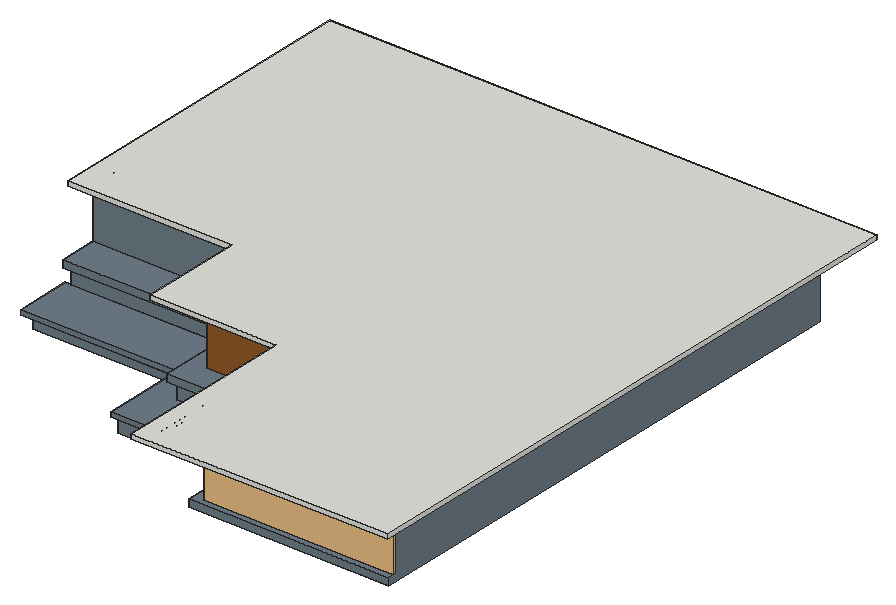
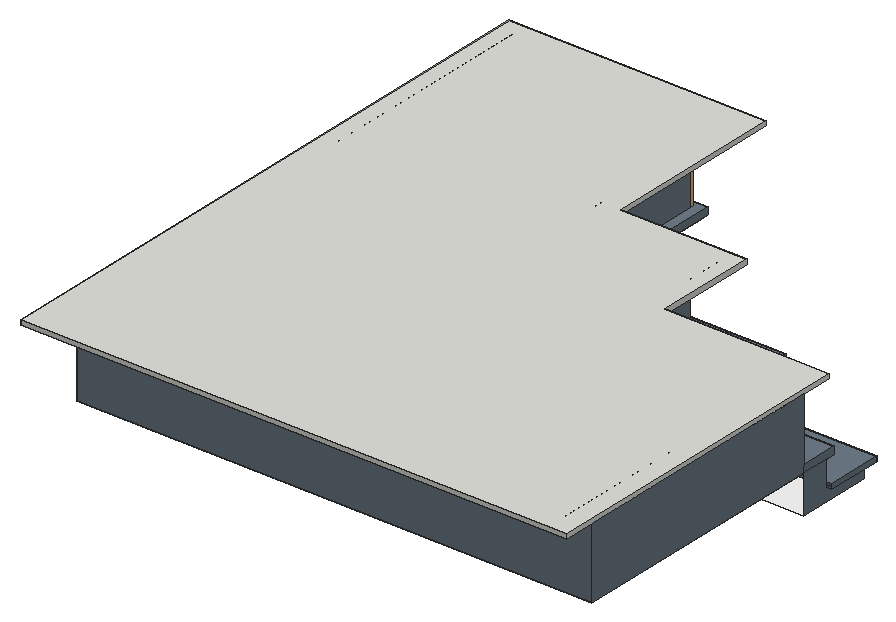
# SketchUp Ruby script. Lengths in inches.
U = 1.inch
M = Sketchup.active_model
def pt(a) = Geom::Point3d.new(a.map { |v| v * U })
def face(e, loops, mat)
  f = e.add_face(loops[0].map { |a| pt(a) })
  loops[1..].each { |l| e.add_face(l.map { |a| pt(a) }).erase! }
  f.material = f.back_material = mat if mat
  f
end
# faces: each face lists its corners as indices into pts; further lists are holes
def faces(e, pts, list, mat = nil) = list.each { |f| face(e, (f[0].is_a?(Array) ? f : [f]).map { |l| l.map { |i| pts[i] } }, mat) }
# xy, xz, yz: faces in a plane at the given z, y or x. An outline is a flat list of corners, or four numbers for a rectangle; further outlines are holes
def ring(l) = l.size == 4 ? [[l[0], l[1]], [l[2], l[1]], [l[2], l[3]], [l[0], l[3]]] : l.each_slice(2).to_a
def flat(e, list, mat, &to3) = list.each { |f| face(e, (f[0].is_a?(Array) ? f : [f]).map { |l| ring(l).map { |u, v| to3.(u, v) } }, mat) }
def xy(e, z, list, mat = nil) = flat(e, list, mat) { |x, y| [x, y, z] }
def xz(e, y, list, mat = nil) = flat(e, list, mat) { |x, z| [x, y, z] }
def yz(e, x, list, mat = nil) = flat(e, list, mat) { |y, z| [x, y, z] }
def lines(e, pts, list) = list.each { |a, b| e.add_line(pt(pts[a]), pt(pts[b])) }
# prism: a flat outline (further loops are holes) pulled along v
def prism(e, loops, v, mat = nil)
  f = face(e, loops, mat); d = Geom::Vector3d.new(v.map { |x| x * U })
  f.pushpull(f.normal.samedirection?(d) ? d.length : -d.length)
end
def box(e, o, s, mat = nil) = prism(e, [[o, [o[0] + s[0], o[1], o[2]], [o[0] + s[0], o[1] + s[1], o[2]], [o[0], o[1] + s[1], o[2]]]], [0, 0, s[2]], mat)
def at(x, y, z, deg = 0) = Geom::Transformation.translation(pt([x, y, z])) * Geom::Transformation.rotation(ORIGIN, Z_AXIS, deg.degrees)
def axes(o, x, y, z) = Geom::Transformation.new([*x, 0, *y, 0, *z, 0, *pt(o).to_a, 1])
def part(name) = M.definitions.add(name)
# library, detail: a bought-in or finely detailed component or shape, given as its bounding box
def library(name, o, s) = part(name).tap { |d| box(d.entities, o, s) }
def detail(e, o, s) = box(e.add_group.entities, o, s)
def put(e, d, t, mat = nil) = e.add_instance(d, t).tap { |i| i.material = mat if mat }
def group(e, t, mat = nil) = e.add_group.tap { |g| g.transformation = t; g.material = mat if mat }.entities
root = M.entities
M.materials.add("Heather_Cuffs").color = [111, 126, 137]
M.materials.add("[Color E05]").color = [255, 255, 0]
M.materials.add("[Color M00]").color = [255, 255, 255]
M.materials.add("[Color M01]").color = [226, 226, 226]
M.materials.add("[Wood Cherry Original]").color = [152, 86, 42]
M.materials.add("[Wood Floor Parquet]").color = [145, 89, 39]
M.materials.add("termopan").color = [253, 253, 253]
c1 = library("Fence panel",[0,-3,0],[162,3,54])
xy(root,330,[[490.93,297.91,490.15,298.01,489.43,298.31,488.81,298.79,488.33,299.41,488.03,300.13,487.93,300.91,488.03,301.68,488.33,302.41,488.81,303.03,489.43,303.5,490.15,303.8,490.93,303.91,491.71,303.8,492.43,303.5,493.05,303.03,493.53,302.41,493.83,301.68,493.93,300.91,493.83,300.13,493.53,299.41,493.05,298.79,492.43,298.31,491.71,298.01],[406.58,298.81,405.81,298.91,405.08,299.21,404.46,299.69,403.98,300.31,403.69,301.03,403.58,301.81,403.69,302.58,403.98,303.31,404.46,303.93,405.08,304.4,405.81,304.7,406.58,304.81,407.36,304.7,408.08,304.4,408.7,303.93,409.18,303.31,409.48,302.58,409.58,301.81,409.48,301.03,409.18,300.31,408.7,299.69,408.08,299.21,407.36,298.91],[300.21,365.29,299.43,365.39,298.71,365.69,298.09,366.17,297.61,366.79,297.3125,367.52,297.21,368.29,297.3125,369.07,297.61,369.79,298.09,370.41,298.71,370.89,299.43,371.19,300.21,371.29,300.99,371.19,301.71,370.89,302.33,370.41,302.81,369.79,303.11,369.07,303.21,368.29,303.11,367.52,302.81,366.79,302.33,366.17,301.71,365.69,300.99,365.39],[338.49,366.3,337.71,366.4,336.99,366.7,336.37,367.18,335.89,367.8,335.59,368.52,335.49,369.3,335.59,370.08,335.89,370.8,336.37,371.42,336.99,371.9,337.71,372.2,338.49,372.3,339.27,372.2,339.99,371.9,340.61,371.42,341.09,370.8,341.39,370.08,341.49,369.3,341.39,368.52,341.09,367.8,340.61,367.18,339.99,366.7,339.27,366.4],[372.37,366.74,371.59,366.84,370.87,367.14,370.25,367.62,369.77,368.24,369.47,368.96,369.37,369.74,369.47,370.51,369.77,371.24,370.25,371.86,370.87,372.34,371.59,372.63,372.37,372.74,373.15,372.63,373.87,372.34,374.49,371.86,374.97,371.24,375.27,370.51,375.37,369.74,375.27,368.96,374.97,368.24,374.49,367.62,373.87,367.14,373.15,366.84]],"[Color E05]")
xy(root,331,[[[395.22,281.96,395.22,356.89,262.22,356.89,262.22,420.96,429.22,420.96,429.22,333.96,540.22,333.96,540.22,281.96],[490.93,297.91,491.71,298.01,492.43,298.31,493.05,298.79,493.53,299.41,493.83,300.13,493.93,300.91,493.83,301.68,493.53,302.41,493.05,303.03,492.43,303.5,491.71,303.8,490.93,303.91,490.15,303.8,489.43,303.5,488.81,303.03,488.33,302.41,488.03,301.68,487.93,300.91,488.03,300.13,488.33,299.41,488.81,298.79,489.43,298.31,490.15,298.01],[300.21,365.29,300.99,365.39,301.71,365.69,302.33,366.17,302.81,366.79,303.11,367.52,303.21,368.29,303.11,369.07,302.81,369.79,302.33,370.41,301.71,370.89,300.99,371.19,300.21,371.29,299.43,371.19,298.71,370.89,298.09,370.41,297.61,369.79,297.3125,369.07,297.21,368.29,297.3125,367.52,297.61,366.79,298.09,366.17,298.71,365.69,299.43,365.39],[338.49,366.3,339.27,366.4,339.99,366.7,340.61,367.18,341.09,367.8,341.39,368.52,341.49,369.3,341.39,370.08,341.09,370.8,340.61,371.42,339.99,371.9,339.27,372.2,338.49,372.3,337.71,372.2,336.99,371.9,336.37,371.42,335.89,370.8,335.59,370.08,335.49,369.3,335.59,368.52,335.89,367.8,336.37,367.18,336.99,366.7,337.71,366.4],[372.37,366.74,373.15,366.84,373.87,367.14,374.49,367.62,374.97,368.24,375.27,368.96,375.37,369.74,375.27,370.51,374.97,371.24,374.49,371.86,373.87,372.34,373.15,372.63,372.37,372.74,371.59,372.63,370.87,372.34,370.25,371.86,369.77,371.24,369.47,370.51,369.37,369.74,369.47,368.96,369.77,368.24,370.25,367.62,370.87,367.14,371.59,366.84],[406.58,298.81,407.36,298.91,408.08,299.21,408.7,299.69,409.18,300.31,409.48,301.03,409.58,301.81,409.48,302.58,409.18,303.31,408.7,303.93,408.08,304.4,407.36,304.7,406.58,304.81,405.81,304.7,405.08,304.4,404.46,303.93,403.98,303.31,403.69,302.58,403.58,301.81,403.69,301.03,403.98,300.31,404.46,299.69,405.08,299.21,405.81,298.91]]],"termopan")
xy(root,343,[[391.22,278.96,415.22,281.96],[415.22,278.96,540.22,281.96],[391.22,281.96,395.22,319.96],[395.22,281.96,415.22,319.96],[415.22,281.96,540.22,319.96],
  [395.22,319.96,415.22,319.96,415.22,397.89,413.22,397.89,413.22,395.89,262.22,395.89,262.22,356.89,395.22,356.89],[391.22,319.96,395.22,356.89],[257.22,349.89,262.22,395.89],[262.22,349.89,391.22,356.89],[257.22,395.89,262.22,397.89],
  [262.22,395.89,402.22,397.89],[402.22,395.89,413.22,397.89]],"Heather_Cuffs")
xy(root,347,[[391.22,278.96,540.22,278.96,540.22,319.96,415.22,319.96,415.22,397.89,257.22,397.89,257.22,349.89,391.22,349.89]],"Heather_Cuffs")
xy(root,363.8,[[531.22,186.96,702.22,194.96],[[540.22,194.96,702.22,194.96,702.22,646.96,262.22,646.96,262.22,397.89,415.22,397.89,415.22,319.96,540.22,319.96],[549.22,203.96,549.22,342.96,438.22,342.96,438.22,429.96,271.22,429.96,271.22,637.96,693.22,637.96,693.22,203.96]],[531.22,194.96,540.22,278.96],[531.22,278.96,540.22,281.96],[531.22,281.96,540.22,319.96],
  [413.22,310.96,531.22,319.96],[413.22,319.96,415.22,397.89],[262.22,388.89,402.22,397.89],[402.22,388.89,413.22,397.89]],"Heather_Cuffs")
xy(root,370,[[531.22,186.96,702.22,186.96,702.22,194.96,540.22,194.96,540.22,333.96,429.22,333.96,429.22,420.96,262.22,420.96,262.22,388.89,413.22,388.89,413.22,310.96,531.22,310.96],[438.22,342.96,438.35,420.96]],"Heather_Cuffs")
xy(root,424,[[540.22,194.96,702.22,194.96,702.22,646.96,262.22,646.96,262.22,420.96,429.22,420.96,429.22,333.96,549.22,333.96,549.22,342.96,438.35,342.96,438.35,420.96,438.22,420.96,438.22,429.96,271.22,429.96,271.22,637.96,693.22,637.96,693.22,203.96,549.22,203.96,549.22,333.96,540.22,333.96]],"Heather_Cuffs")
xy(root,424,[[[510.22,151.96,510.22,306.96,402.22,306.96,402.22,393.96,262.22,393.96,262.22,673.96,729.22,673.96,729.22,151.96],[523.35,165.08,716.09,165.08,716.09,660.83,275.35,660.83,275.35,407.08,415.35,407.08,415.35,320.08,523.35,320.08]],[526.88,168.61,526.88,323.61,418.88,323.61,418.88,410.61,278.88,410.61,278.88,657.3,712.5625,657.3,712.5625,168.61]],"[Wood Cherry Original]")
xy(root,427,[[[523.35,165.08,523.35,320.08,415.35,320.08,415.35,407.08,275.35,407.08,275.35,660.83,716.09,660.83,716.09,165.08],[526.88,168.61,712.5625,168.61,712.5625,657.3,278.88,657.3,278.88,410.61,418.88,410.61,418.88,323.61,526.88,323.61]]],"[Color E05]")
xy(root,428,[[510.22,151.96,729.22,151.96,729.22,673.96,262.22,673.96,262.22,393.96,402.22,393.96,402.22,306.96,510.22,306.96]])
xz(root,151.96,[[510.22,424,729.22,428]])
xz(root,165.08,[[523.35,424,716.09,427]])
xz(root,168.61,[[526.88,424,712.5625,427]])
xz(root,186.96,[[531.22,363.8,702.22,370]],"Heather_Cuffs")
xz(root,194.96,[[543.35,370,693.22,424],[693.22,370,702.22,424]],"Heather_Cuffs")
xz(root,203.96,[[549.22,363.8,693.22,424]],"Heather_Cuffs")
xz(root,278.96,[[391.22,343,540.22,347]],"Heather_Cuffs")
xz(root,281.96,[[395.22,331,540.22,343]],"Heather_Cuffs")
xz(root,306.96,[[402.22,424,510.22,428]])
xz(root,310.96,[[413.22,363.8,531.22,370]],"Heather_Cuffs")
xz(root,319.96,[[415.22,343,540.22,347],[415.22,347,540.22,363.8]],"Heather_Cuffs")
xz(root,320.08,[[415.35,424,523.35,427]])
xz(root,323.61,[[418.88,424,526.88,427]])
xz(root,333.96,[[540.22,370,540.22,424,549.22,424]],"Heather_Cuffs")
xz(root,333.96,[[429.22,370,540.22,424]],"[Wood Floor Parquet]")
xz(root,342.96,[[438.22,363.8,438.22,370,438.35,370,438.35,424,549.22,424,549.22,363.8]],"Heather_Cuffs")
xz(root,349.89,[[257.22,343,391.22,347]],"Heather_Cuffs")
xz(root,356.89,[[262.22,331,395.22,343]],"Heather_Cuffs")
xz(root,388.89,[[262.22,363.8,413.22,370]],"Heather_Cuffs")
xz(root,393.96,[[262.22,424,402.22,428]])
xz(root,397.89,[[257.22,343,262.22,345],[262.22,343,402.22,347],[402.22,343,413.22,347],[413.22,343,415.22,347],[257.22,345,262.22,347],
  [262.22,347,402.22,363.8],[402.22,347,413.22,363.8],[413.22,347,415.22,363.8]],"Heather_Cuffs")
xz(root,407.08,[[275.35,424,415.35,427]])
xz(root,410.61,[[278.88,424,418.88,427]])
xz(root,420.96,[[262.22,370,429.22,424],[438.22,370,438.35,424]],"Heather_Cuffs")
xz(root,429.96,[[271.22,363.8,438.22,424]],"Heather_Cuffs")
xz(root,637.96,[[271.22,363.8,693.22,424]],"Heather_Cuffs")
xz(root,646.96,[[262.22,363.8,702.22,424]],"Heather_Cuffs")
xz(root,657.3,[[278.88,424,712.5625,427]])
xz(root,660.83,[[275.35,424,716.09,427]])
xz(root,673.96,[[262.22,424,729.22,428]])
yz(root,257.22,[[349.89,343,397.89,347]],"Heather_Cuffs")
yz(root,262.22,[[393.96,424,673.96,428]])
yz(root,262.22,[[356.89,331,356.89,343,397.89,343,397.89,363.8,420.96,363.8,420.96,331],[388.89,363.8,420.96,370],[420.96,363.8,646.96,424]],"Heather_Cuffs")
yz(root,271.22,[[429.96,363.8,637.96,424]],"Heather_Cuffs")
yz(root,275.35,[[407.08,424,660.83,427]])
yz(root,278.88,[[410.61,424,657.3,427]])
yz(root,391.22,[[278.96,343,349.89,347]],"Heather_Cuffs")
yz(root,395.22,[[281.96,331,356.89,343]],"Heather_Cuffs")
yz(root,402.22,[[306.96,424,393.96,428]])
yz(root,413.22,[[395.89,343,397.89,345],[310.96,363.8,388.89,370]],"Heather_Cuffs")
yz(root,415.22,[[319.96,343,397.89,347],[319.96,347,397.89,363.8]],"Heather_Cuffs")
yz(root,415.35,[[320.08,424,407.08,427]])
yz(root,418.88,[[323.61,424,410.61,427]])
yz(root,429.22,[[333.96,370,420.96,424]],"Heather_Cuffs")
yz(root,438.22,[[342.96,363.8,429.96,363.8,429.96,424,420.96,424,420.96,370,342.96,370]],"Heather_Cuffs")
yz(root,438.35,[[342.96,370,420.96,424]],"Heather_Cuffs")
yz(root,510.22,[[151.96,424,306.96,428]])
yz(root,523.35,[[165.08,424,320.08,427]])
yz(root,526.88,[[168.61,424,323.61,427]])
yz(root,531.22,[[186.96,363.8,310.96,370]],"Heather_Cuffs")
yz(root,540.22,[[278.96,343,281.96,347],[281.96,343,319.96,347],[278.96,347,281.96,363.8],[281.96,347,319.96,363.8],[194.96,370,333.96,424]],"Heather_Cuffs")
yz(root,549.22,[[203.96,363.8,342.96,424]],"Heather_Cuffs")
yz(root,693.22,[[203.96,363.8,637.96,424]],"Heather_Cuffs")
yz(root,702.22,[[186.96,363.8,646.96,363.8,646.96,424,194.96,424,194.96,370,186.96,370]],"Heather_Cuffs")
yz(root,712.5625,[[168.61,424,657.3,427]])
yz(root,716.09,[[165.08,424,660.83,427]])
yz(root,729.22,[[151.96,424,673.96,428]])
p = [[490.93,297.91,331],[490.15,298.01,331],[490.15,298.01,330],[490.93,297.91,330],[491.71,298.01,331],[491.71,298.01,330],
  [489.43,298.31,331],[489.43,298.31,330],[492.43,298.31,331],[492.43,298.31,330],[488.81,298.79,331],[488.81,298.79,330],
  [493.05,298.79,331],[493.05,298.79,330],[406.58,298.81,331],[405.81,298.91,331],[405.81,298.91,330],[406.58,298.81,330],
  [407.36,298.91,331],[407.36,298.91,330],[488.33,299.41,331],[488.33,299.41,330],[493.53,299.41,331],[493.53,299.41,330],
  [405.08,299.21,331],[405.08,299.21,330],[408.08,299.21,331],[408.08,299.21,330],[404.46,299.69,331],[404.46,299.69,330],
  [408.7,299.69,331],[408.7,299.69,330],[488.03,300.13,331],[488.03,300.13,330],[493.83,300.13,331],[493.83,300.13,330],
  [403.98,300.31,331],[403.98,300.31,330],[409.18,300.31,331],[409.18,300.31,330],[487.93,300.91,331],[487.93,300.91,330],
  [493.93,300.91,331],[493.93,300.91,330],[403.69,301.03,331],[403.69,301.03,330],[409.48,301.03,331],[409.48,301.03,330],
  [488.03,301.68,331],[488.03,301.68,330],[493.83,301.68,331],[493.83,301.68,330],[403.58,301.81,331],[403.58,301.81,330],
  [409.58,301.81,331],[409.58,301.81,330],[488.33,302.41,331],[488.33,302.41,330],[493.53,302.41,331],[493.53,302.41,330],
  [403.69,302.58,331],[403.69,302.58,330],[409.48,302.58,331],[409.48,302.58,330],[488.81,303.03,331],[488.81,303.03,330],
  [493.05,303.03,331],[493.05,303.03,330],[403.98,303.31,331],[403.98,303.31,330],[409.18,303.31,331],[409.18,303.31,330],
  [489.43,303.5,331],[489.43,303.5,330],[492.43,303.5,331],[492.43,303.5,330],[404.46,303.93,331],[404.46,303.93,330],
  [408.7,303.93,331],[408.7,303.93,330],[490.15,303.8,331],[490.15,303.8,330],[491.71,303.8,331],[491.71,303.8,330],
  [490.93,303.91,331],[490.93,303.91,330],[405.08,304.4,331],[405.08,304.4,330],[408.08,304.4,331],[408.08,304.4,330],
  [405.81,304.7,331],[405.81,304.7,330],[407.36,304.7,331],[407.36,304.7,330],[406.58,304.81,331],[406.58,304.81,330],
  [300.21,365.29,331],[299.43,365.39,331],[299.43,365.39,330],[300.21,365.29,330],[300.99,365.39,331],[300.99,365.39,330],
  [298.71,365.69,331],[298.71,365.69,330],[301.71,365.69,331],[301.71,365.69,330],[298.09,366.17,331],[298.09,366.17,330],
  [302.33,366.17,331],[302.33,366.17,330],[297.61,366.79,331],[297.61,366.79,330],[302.81,366.79,331],[302.81,366.79,330],
  [338.49,366.3,331],[337.71,366.4,331],[337.71,366.4,330],[338.49,366.3,330],[339.27,366.4,331],[339.27,366.4,330],
  [336.99,366.7,331],[336.99,366.7,330],[339.99,366.7,331],[339.99,366.7,330],[336.37,367.18,331],[336.37,367.18,330],
  [340.61,367.18,331],[340.61,367.18,330],[372.37,366.74,331],[371.59,366.84,331],[371.59,366.84,330],[372.37,366.74,330],
  [373.15,366.84,331],[373.15,366.84,330],[297.3125,367.52,331],[297.3125,367.52,330],[303.11,367.52,331],[303.11,367.52,330],
  [370.87,367.14,331],[370.87,367.14,330],[373.87,367.14,331],[373.87,367.14,330],[370.25,367.62,331],[370.25,367.62,330],
  [374.49,367.62,331],[374.49,367.62,330],[335.89,367.8,331],[335.89,367.8,330],[341.09,367.8,331],[341.09,367.8,330],
  [297.21,368.29,331],[297.21,368.29,330],[303.21,368.29,331],[303.21,368.29,330],[369.77,368.24,331],[369.77,368.24,330],
  [374.97,368.24,331],[374.97,368.24,330],[335.59,368.52,331],[335.59,368.52,330],[341.39,368.52,331],[341.39,368.52,330],
  [369.47,368.96,331],[369.47,368.96,330],[375.27,368.96,331],[375.27,368.96,330],[297.3125,369.07,331],[297.3125,369.07,330],
  [303.11,369.07,331],[303.11,369.07,330],[335.49,369.3,331],[335.49,369.3,330],[341.49,369.3,331],[341.49,369.3,330],
  [369.37,369.74,331],[369.37,369.74,330],[375.37,369.74,331],[375.37,369.74,330],[297.61,369.79,331],[297.61,369.79,330],
  [302.81,369.79,331],[302.81,369.79,330],[335.59,370.08,331],[335.59,370.08,330],[341.39,370.08,331],[341.39,370.08,330],
  [369.47,370.51,331],[369.47,370.51,330],[375.27,370.51,331],[375.27,370.51,330],[298.09,370.41,331],[298.09,370.41,330],
  [302.33,370.41,331],[302.33,370.41,330],[335.89,370.8,331],[335.89,370.8,330],[341.09,370.8,331],[341.09,370.8,330],
  [298.71,370.89,331],[298.71,370.89,330],[301.71,370.89,331],[301.71,370.89,330],[369.77,371.24,331],[369.77,371.24,330],
  [374.97,371.24,331],[374.97,371.24,330],[336.37,371.42,331],[336.37,371.42,330],[340.61,371.42,331],[340.61,371.42,330],
  [299.43,371.19,331],[299.43,371.19,330],[300.99,371.19,331],[300.99,371.19,330],[300.21,371.29,331],[300.21,371.29,330],
  [370.25,371.86,331],[370.25,371.86,330],[374.49,371.86,331],[374.49,371.86,330],[336.99,371.9,331],[336.99,371.9,330],
  [339.99,371.9,331],[339.99,371.9,330],[337.71,372.2,331],[337.71,372.2,330],[339.27,372.2,331],[339.27,372.2,330],
  [370.87,372.34,331],[370.87,372.34,330],[373.87,372.34,331],[373.87,372.34,330],[338.49,372.3,331],[338.49,372.3,330],
  [371.59,372.63,331],[371.59,372.63,330],[373.15,372.63,331],[373.15,372.63,330],[372.37,372.74,331],[372.37,372.74,330],
  [413.22,395.89,345],[262.22,395.89,345],[415.22,319.96,345],[395.22,319.96,345]]
faces(root,p,[[0,1,2,3],[4,0,3,5],[1,6,7,2],[8,4,5,9],[6,10,11,7],[12,8,9,13],[14,15,16,17],[18,14,17,19],
  [10,20,21,11],[22,12,13,23],[15,24,25,16],[26,18,19,27],[24,28,29,25],[30,26,27,31],[20,32,33,21],[34,22,23,35],
  [28,36,37,29],[38,30,31,39],[32,40,41,33],[42,34,35,43],[36,44,45,37],[46,38,39,47],[40,48,49,41],[50,42,43,51],
  [44,52,53,45],[54,46,47,55],[48,56,57,49],[58,50,51,59],[52,60,61,53],[62,54,55,63],[56,64,65,57],[66,58,59,67],
  [60,68,69,61],[70,62,63,71],[64,72,73,65],[74,66,67,75],[68,76,77,69],[78,70,71,79],[72,80,81,73],[82,74,75,83],
  [80,84,85,81],[84,82,83,85],[76,86,87,77],[88,78,79,89],[86,90,91,87],[92,88,89,93],[90,94,95,91],[94,92,93,95],
  [96,97,98,99],[100,96,99,101],[97,102,103,98],[104,100,101,105],[102,106,107,103],[108,104,105,109],[106,110,111,107],[112,108,109,113],
  [114,115,116,117],[118,114,117,119],[115,120,121,116],[122,118,119,123],[120,124,125,121],[126,122,123,127],[128,129,130,131],[132,128,131,133],
  [110,134,135,111],[136,112,113,137],[129,138,139,130],[140,132,133,141],[138,142,143,139],[144,140,141,145],[124,146,147,125],[148,126,127,149],
  [134,150,151,135],[152,136,137,153],[142,154,155,143],[156,144,145,157],[146,158,159,147],[160,148,149,161],[154,162,163,155],[164,156,157,165],
  [150,166,167,151],[168,152,153,169],[158,170,171,159],[172,160,161,173],[162,174,175,163],[176,164,165,177],[166,178,179,167],[180,168,169,181],
  [170,182,183,171],[184,172,173,185],[174,186,187,175],[188,176,177,189],[178,190,191,179],[192,180,181,193],[182,194,195,183],[196,184,185,197],
  [190,198,199,191],[200,192,193,201],[186,202,203,187],[204,188,189,205],[194,206,207,195],[208,196,197,209],[198,210,211,199],[212,200,201,213],
  [210,214,215,211],[214,212,213,215],[202,216,217,203],[218,204,205,219],[206,220,221,207],[222,208,209,223],[220,224,225,221],[226,222,223,227],
  [216,228,229,217],[230,218,219,231],[224,232,233,225],[232,226,227,233],[228,234,235,229],[236,230,231,237],[234,238,239,235],[238,236,237,239]],"termopan")
lines(root,p,[[240,241],[242,243]])
put(root,c1,at(540.22,194.96,370),"Heather_Cuffs")
g1 = group(root,at(296.91,399.6,424))
xy(g1,-1,[[-2,0,-2.52,0.07,-3,0.27,-3.41,0.59,-3.73,1,-3.93,1.48,-4,2,-3.93,2.52,-3.73,3,-3.41,3.41,-3,3.73,-2.52,3.93,-2,4,-1.48,3.93,-1,3.73,-0.59,3.41,-0.27,3,-0.07,2.52,0,2,-0.07,1.48,-0.27,1,-0.59,0.59,-1,0.27,-1.48,0.07]],"[Color E05]")
xy(g1,0,[[-2,0,-1.48,0.07,-1,0.27,-0.59,0.59,-0.27,1,-0.07,1.48,0,2,-0.07,2.52,-0.27,3,-0.59,3.41,-1,3.73,-1.48,3.93,-2,4,-2.52,3.93,-3,3.73,-3.41,3.41,-3.73,3,-3.93,2.52,-4,2,-3.93,1.48,-3.73,1,-3.41,0.59,-3,0.27,-2.52,0.07]],"[Wood Cherry Original]")
p = [[-2,0,0],[-2.52,0.07,0],[-2.52,0.07,-1],[-2,0,-1],[-1.48,0.07,0],[-1.48,0.07,-1],
  [-3,0.27,0],[-3,0.27,-1],[-1,0.27,0],[-1,0.27,-1],[-3.41,0.59,0],[-3.41,0.59,-1],
  [-0.59,0.59,0],[-0.59,0.59,-1],[-3.73,1,0],[-3.73,1,-1],[-0.27,1,0],[-0.27,1,-1],
  [-3.93,1.48,0],[-3.93,1.48,-1],[-0.07,1.48,0],[-0.07,1.48,-1],[-4,2,0],[-4,2,-1],
  [0,2,0],[0,2,-1],[-3.93,2.52,0],[-3.93,2.52,-1],[-0.07,2.52,0],[-0.07,2.52,-1],
  [-3.73,3,0],[-3.73,3,-1],[-0.27,3,0],[-0.27,3,-1],[-3.41,3.41,0],[-3.41,3.41,-1],
  [-0.59,3.41,0],[-0.59,3.41,-1],[-3,3.73,0],[-3,3.73,-1],[-1,3.73,0],[-1,3.73,-1],
  [-2.52,3.93,0],[-2.52,3.93,-1],[-1.48,3.93,0],[-1.48,3.93,-1],[-2,4,0],[-2,4,-1]]
faces(g1,p,[[0,1,2,3],[4,0,3,5],[1,6,7,2],[8,4,5,9],[6,10,11,7],[12,8,9,13],[10,14,15,11],[16,12,13,17],
  [14,18,19,15],[20,16,17,21],[18,22,23,19],[24,20,21,25],[22,26,27,23],[28,24,25,29],[26,30,31,27],[32,28,29,33],
  [30,34,35,31],[36,32,33,37],[34,38,39,35],[40,36,37,41],[38,42,43,39],[44,40,41,45],[42,46,47,43],[46,44,45,47]],"[Color M00]")
g2 = group(root,at(334.91,399.6,424))
xy(g2,-1,[[-2,0,-2.52,0.07,-3,0.27,-3.41,0.59,-3.73,1,-3.93,1.48,-4,2,-3.93,2.52,-3.73,3,-3.41,3.41,-3,3.73,-2.52,3.93,-2,4,-1.48,3.93,-1,3.73,-0.59,3.41,-0.27,3,-0.07,2.52,0,2,-0.07,1.48,-0.27,1,-0.59,0.59,-1,0.27,-1.48,0.07]],"[Color E05]")
xy(g2,0,[[-2,0,-1.48,0.07,-1,0.27,-0.59,0.59,-0.27,1,-0.07,1.48,0,2,-0.07,2.52,-0.27,3,-0.59,3.41,-1,3.73,-1.48,3.93,-2,4,-2.52,3.93,-3,3.73,-3.41,3.41,-3.73,3,-3.93,2.52,-4,2,-3.93,1.48,-3.73,1,-3.41,0.59,-3,0.27,-2.52,0.07]],"[Wood Cherry Original]")
p = [[-2,0,0],[-2.52,0.07,0],[-2.52,0.07,-1],[-2,0,-1],[-1.48,0.07,0],[-1.48,0.07,-1],
  [-3,0.27,0],[-3,0.27,-1],[-1,0.27,0],[-1,0.27,-1],[-3.41,0.59,0],[-3.41,0.59,-1],
  [-0.59,0.59,0],[-0.59,0.59,-1],[-3.73,1,0],[-3.73,1,-1],[-0.27,1,0],[-0.27,1,-1],
  [-3.93,1.48,0],[-3.93,1.48,-1],[-0.07,1.48,0],[-0.07,1.48,-1],[-4,2,0],[-4,2,-1],
  [0,2,0],[0,2,-1],[-3.93,2.52,0],[-3.93,2.52,-1],[-0.07,2.52,0],[-0.07,2.52,-1],
  [-3.73,3,0],[-3.73,3,-1],[-0.27,3,0],[-0.27,3,-1],[-3.41,3.41,0],[-3.41,3.41,-1],
  [-0.59,3.41,0],[-0.59,3.41,-1],[-3,3.73,0],[-3,3.73,-1],[-1,3.73,0],[-1,3.73,-1],
  [-2.52,3.93,0],[-2.52,3.93,-1],[-1.48,3.93,0],[-1.48,3.93,-1],[-2,4,0],[-2,4,-1]]
faces(g2,p,[[0,1,2,3],[4,0,3,5],[1,6,7,2],[8,4,5,9],[6,10,11,7],[12,8,9,13],[10,14,15,11],[16,12,13,17],
  [14,18,19,15],[20,16,17,21],[18,22,23,19],[24,20,21,25],[22,26,27,23],[28,24,25,29],[26,30,31,27],[32,28,29,33],
  [30,34,35,31],[36,32,33,37],[34,38,39,35],[40,36,37,41],[38,42,43,39],[44,40,41,45],[42,46,47,43],[46,44,45,47]],"[Color M00]")
g3 = group(root,at(378.91,399.6,424))
prism(g3,[[[-1.48,3.93,-1],[-1,3.73,-1],[-0.59,3.41,-1],[-0.27,3,-1],[-0.07,2.52,-1],[0,2,-1],[-0.07,1.48,-1],[-0.27,1,-1],[-0.59,0.59,-1],[-1,0.27,-1],[-1.48,0.07,-1],[-2,0,-1],[-2.52,0.07,-1],[-3,0.27,-1],[-3.41,0.59,-1],[-3.73,1,-1],[-3.93,1.48,-1],[-4,2,-1],[-3.93,2.52,-1],[-3.73,3,-1],[-3.41,3.41,-1],[-3,3.73,-1],[-2.52,3.93,-1],[-2,4,-1]]],[0,0,1],"[Wood Cherry Original]")
g4 = group(root,at(412.91,399.6,424))
xy(g4,-1,[[-2,0,-2.52,0.07,-3,0.27,-3.41,0.59,-3.73,1,-3.93,1.48,-4,2,-3.93,2.52,-3.73,3,-3.41,3.41,-3,3.73,-2.52,3.93,-2,4,-1.48,3.93,-1,3.73,-0.59,3.41,-0.27,3,-0.07,2.52,0,2,-0.07,1.48,-0.27,1,-0.59,0.59,-1,0.27,-1.48,0.07]],"[Color E05]")
xy(g4,0,[[-2,0,-1.48,0.07,-1,0.27,-0.59,0.59,-0.27,1,-0.07,1.48,0,2,-0.07,2.52,-0.27,3,-0.59,3.41,-1,3.73,-1.48,3.93,-2,4,-2.52,3.93,-3,3.73,-3.41,3.41,-3.73,3,-3.93,2.52,-4,2,-3.93,1.48,-3.73,1,-3.41,0.59,-3,0.27,-2.52,0.07]],"[Wood Cherry Original]")
p = [[-2,0,0],[-2.52,0.07,0],[-2.52,0.07,-1],[-2,0,-1],[-1.48,0.07,0],[-1.48,0.07,-1],
  [-3,0.27,0],[-3,0.27,-1],[-1,0.27,0],[-1,0.27,-1],[-3.41,0.59,0],[-3.41,0.59,-1],
  [-0.59,0.59,0],[-0.59,0.59,-1],[-3.73,1,0],[-3.73,1,-1],[-0.27,1,0],[-0.27,1,-1],
  [-3.93,1.48,0],[-3.93,1.48,-1],[-0.07,1.48,0],[-0.07,1.48,-1],[-4,2,0],[-4,2,-1],
  [0,2,0],[0,2,-1],[-3.93,2.52,0],[-3.93,2.52,-1],[-0.07,2.52,0],[-0.07,2.52,-1],
  [-3.73,3,0],[-3.73,3,-1],[-0.27,3,0],[-0.27,3,-1],[-3.41,3.41,0],[-3.41,3.41,-1],
  [-0.59,3.41,0],[-0.59,3.41,-1],[-3,3.73,0],[-3,3.73,-1],[-1,3.73,0],[-1,3.73,-1],
  [-2.52,3.93,0],[-2.52,3.93,-1],[-1.48,3.93,0],[-1.48,3.93,-1],[-2,4,0],[-2,4,-1]]
faces(g4,p,[[0,1,2,3],[4,0,3,5],[1,6,7,2],[8,4,5,9],[6,10,11,7],[12,8,9,13],[10,14,15,11],[16,12,13,17],
  [14,18,19,15],[20,16,17,21],[18,22,23,19],[24,20,21,25],[22,26,27,23],[28,24,25,29],[26,30,31,27],[32,28,29,33],
  [30,34,35,31],[36,32,33,37],[34,38,39,35],[40,36,37,41],[38,42,43,39],[44,40,41,45],[42,46,47,43],[46,44,45,47]],"[Color M00]")
g5 = group(root,at(412.91,355.6,424))
xy(g5,-1,[[-2,0,-2.52,0.07,-3,0.27,-3.41,0.59,-3.73,1,-3.93,1.48,-4,2,-3.93,2.52,-3.73,3,-3.41,3.41,-3,3.73,-2.52,3.93,-2,4,-1.48,3.93,-1,3.73,-0.59,3.41,-0.27,3,-0.07,2.52,0,2,-0.07,1.48,-0.27,1,-0.59,0.59,-1,0.27,-1.48,0.07]],"[Color E05]")
xy(g5,0,[[-2,0,-1.48,0.07,-1,0.27,-0.59,0.59,-0.27,1,-0.07,1.48,0,2,-0.07,2.52,-0.27,3,-0.59,3.41,-1,3.73,-1.48,3.93,-2,4,-2.52,3.93,-3,3.73,-3.41,3.41,-3.73,3,-3.93,2.52,-4,2,-3.93,1.48,-3.73,1,-3.41,0.59,-3,0.27,-2.52,0.07]],"[Wood Cherry Original]")
p = [[-2,0,0],[-2.52,0.07,0],[-2.52,0.07,-1],[-2,0,-1],[-1.48,0.07,0],[-1.48,0.07,-1],
  [-3,0.27,0],[-3,0.27,-1],[-1,0.27,0],[-1,0.27,-1],[-3.41,0.59,0],[-3.41,0.59,-1],
  [-0.59,0.59,0],[-0.59,0.59,-1],[-3.73,1,0],[-3.73,1,-1],[-0.27,1,0],[-0.27,1,-1],
  [-3.93,1.48,0],[-3.93,1.48,-1],[-0.07,1.48,0],[-0.07,1.48,-1],[-4,2,0],[-4,2,-1],
  [0,2,0],[0,2,-1],[-3.93,2.52,0],[-3.93,2.52,-1],[-0.07,2.52,0],[-0.07,2.52,-1],
  [-3.73,3,0],[-3.73,3,-1],[-0.27,3,0],[-0.27,3,-1],[-3.41,3.41,0],[-3.41,3.41,-1],
  [-0.59,3.41,0],[-0.59,3.41,-1],[-3,3.73,0],[-3,3.73,-1],[-1,3.73,0],[-1,3.73,-1],
  [-2.52,3.93,0],[-2.52,3.93,-1],[-1.48,3.93,0],[-1.48,3.93,-1],[-2,4,0],[-2,4,-1]]
faces(g5,p,[[0,1,2,3],[4,0,3,5],[1,6,7,2],[8,4,5,9],[6,10,11,7],[12,8,9,13],[10,14,15,11],[16,12,13,17],
  [14,18,19,15],[20,16,17,21],[18,22,23,19],[24,20,21,25],[22,26,27,23],[28,24,25,29],[26,30,31,27],[32,28,29,33],
  [30,34,35,31],[36,32,33,37],[34,38,39,35],[40,36,37,41],[38,42,43,39],[44,40,41,45],[42,46,47,43],[46,44,45,47]],"[Color M01]")
g6 = group(root,at(412.91,319.6,424))
xy(g6,-1,[[-2,0,-2.52,0.07,-3,0.27,-3.41,0.59,-3.73,1,-3.93,1.48,-4,2,-3.93,2.52,-3.73,3,-3.41,3.41,-3,3.73,-2.52,3.93,-2,4,-1.48,3.93,-1,3.73,-0.59,3.41,-0.27,3,-0.07,2.52,0,2,-0.07,1.48,-0.27,1,-0.59,0.59,-1,0.27,-1.48,0.07]],"[Color E05]")
xy(g6,0,[[-2,0,-1.48,0.07,-1,0.27,-0.59,0.59,-0.27,1,-0.07,1.48,0,2,-0.07,2.52,-0.27,3,-0.59,3.41,-1,3.73,-1.48,3.93,-2,4,-2.52,3.93,-3,3.73,-3.41,3.41,-3.73,3,-3.93,2.52,-4,2,-3.93,1.48,-3.73,1,-3.41,0.59,-3,0.27,-2.52,0.07]],"[Wood Cherry Original]")
p = [[-2,0,0],[-2.52,0.07,0],[-2.52,0.07,-1],[-2,0,-1],[-1.48,0.07,0],[-1.48,0.07,-1],
  [-3,0.27,0],[-3,0.27,-1],[-1,0.27,0],[-1,0.27,-1],[-3.41,0.59,0],[-3.41,0.59,-1],
  [-0.59,0.59,0],[-0.59,0.59,-1],[-3.73,1,0],[-3.73,1,-1],[-0.27,1,0],[-0.27,1,-1],
  [-3.93,1.48,0],[-3.93,1.48,-1],[-0.07,1.48,0],[-0.07,1.48,-1],[-4,2,0],[-4,2,-1],
  [0,2,0],[0,2,-1],[-3.93,2.52,0],[-3.93,2.52,-1],[-0.07,2.52,0],[-0.07,2.52,-1],
  [-3.73,3,0],[-3.73,3,-1],[-0.27,3,0],[-0.27,3,-1],[-3.41,3.41,0],[-3.41,3.41,-1],
  [-0.59,3.41,0],[-0.59,3.41,-1],[-3,3.73,0],[-3,3.73,-1],[-1,3.73,0],[-1,3.73,-1],
  [-2.52,3.93,0],[-2.52,3.93,-1],[-1.48,3.93,0],[-1.48,3.93,-1],[-2,4,0],[-2,4,-1]]
faces(g6,p,[[0,1,2,3],[4,0,3,5],[1,6,7,2],[8,4,5,9],[6,10,11,7],[12,8,9,13],[10,14,15,11],[16,12,13,17],
  [14,18,19,15],[20,16,17,21],[18,22,23,19],[24,20,21,25],[22,26,27,23],[28,24,25,29],[26,30,31,27],[32,28,29,33],
  [30,34,35,31],[36,32,33,37],[34,38,39,35],[40,36,37,41],[38,42,43,39],[44,40,41,45],[42,46,47,43],[46,44,45,47]],"[Color M00]")
g7 = group(root,at(431.86,310.54,424))
xy(g7,-1,[[-2,0,-2.52,0.07,-3,0.27,-3.41,0.59,-3.73,1,-3.93,1.48,-4,2,-3.93,2.52,-3.73,3,-3.41,3.41,-3,3.73,-2.52,3.93,-2,4,-1.48,3.93,-1,3.73,-0.59,3.41,-0.27,3,-0.07,2.52,0,2,-0.07,1.48,-0.27,1,-0.59,0.59,-1,0.27,-1.48,0.07]],"[Color E05]")
xy(g7,0,[[-2,0,-1.48,0.07,-1,0.27,-0.59,0.59,-0.27,1,-0.07,1.48,0,2,-0.07,2.52,-0.27,3,-0.59,3.41,-1,3.73,-1.48,3.93,-2,4,-2.52,3.93,-3,3.73,-3.41,3.41,-3.73,3,-3.93,2.52,-4,2,-3.93,1.48,-3.73,1,-3.41,0.59,-3,0.27,-2.52,0.07]],"[Wood Cherry Original]")
p = [[-2,0,0],[-2.52,0.07,0],[-2.52,0.07,-1],[-2,0,-1],[-1.48,0.07,0],[-1.48,0.07,-1],
  [-3,0.27,0],[-3,0.27,-1],[-1,0.27,0],[-1,0.27,-1],[-3.41,0.59,0],[-3.41,0.59,-1],
  [-0.59,0.59,0],[-0.59,0.59,-1],[-3.73,1,0],[-3.73,1,-1],[-0.27,1,0],[-0.27,1,-1],
  [-3.93,1.48,0],[-3.93,1.48,-1],[-0.07,1.48,0],[-0.07,1.48,-1],[-4,2,0],[-4,2,-1],
  [0,2,0],[0,2,-1],[-3.93,2.52,0],[-3.93,2.52,-1],[-0.07,2.52,0],[-0.07,2.52,-1],
  [-3.73,3,0],[-3.73,3,-1],[-0.27,3,0],[-0.27,3,-1],[-3.41,3.41,0],[-3.41,3.41,-1],
  [-0.59,3.41,0],[-0.59,3.41,-1],[-3,3.73,0],[-3,3.73,-1],[-1,3.73,0],[-1,3.73,-1],
  [-2.52,3.93,0],[-2.52,3.93,-1],[-1.48,3.93,0],[-1.48,3.93,-1],[-2,4,0],[-2,4,-1]]
faces(g7,p,[[0,1,2,3],[4,0,3,5],[1,6,7,2],[8,4,5,9],[6,10,11,7],[12,8,9,13],[10,14,15,11],[16,12,13,17],
  [14,18,19,15],[20,16,17,21],[18,22,23,19],[24,20,21,25],[22,26,27,23],[28,24,25,29],[26,30,31,27],[32,28,29,33],
  [30,34,35,31],[36,32,33,37],[34,38,39,35],[40,36,37,41],[38,42,43,39],[44,40,41,45],[42,46,47,43],[46,44,45,47]],"[Color M00]")
g8 = group(root,at(459.86,310.54,424))
xy(g8,-1,[[-2,0,-2.52,0.07,-3,0.27,-3.41,0.59,-3.73,1,-3.93,1.48,-4,2,-3.93,2.52,-3.73,3,-3.41,3.41,-3,3.73,-2.52,3.93,-2,4,-1.48,3.93,-1,3.73,-0.59,3.41,-0.27,3,-0.07,2.52,0,2,-0.07,1.48,-0.27,1,-0.59,0.59,-1,0.27,-1.48,0.07]],"[Color E05]")
xy(g8,0,[[-2,0,-1.48,0.07,-1,0.27,-0.59,0.59,-0.27,1,-0.07,1.48,0,2,-0.07,2.52,-0.27,3,-0.59,3.41,-1,3.73,-1.48,3.93,-2,4,-2.52,3.93,-3,3.73,-3.41,3.41,-3.73,3,-3.93,2.52,-4,2,-3.93,1.48,-3.73,1,-3.41,0.59,-3,0.27,-2.52,0.07]],"[Wood Cherry Original]")
p = [[-2,0,0],[-2.52,0.07,0],[-2.52,0.07,-1],[-2,0,-1],[-1.48,0.07,0],[-1.48,0.07,-1],
  [-3,0.27,0],[-3,0.27,-1],[-1,0.27,0],[-1,0.27,-1],[-3.41,0.59,0],[-3.41,0.59,-1],
  [-0.59,0.59,0],[-0.59,0.59,-1],[-3.73,1,0],[-3.73,1,-1],[-0.27,1,0],[-0.27,1,-1],
  [-3.93,1.48,0],[-3.93,1.48,-1],[-0.07,1.48,0],[-0.07,1.48,-1],[-4,2,0],[-4,2,-1],
  [0,2,0],[0,2,-1],[-3.93,2.52,0],[-3.93,2.52,-1],[-0.07,2.52,0],[-0.07,2.52,-1],
  [-3.73,3,0],[-3.73,3,-1],[-0.27,3,0],[-0.27,3,-1],[-3.41,3.41,0],[-3.41,3.41,-1],
  [-0.59,3.41,0],[-0.59,3.41,-1],[-3,3.73,0],[-3,3.73,-1],[-1,3.73,0],[-1,3.73,-1],
  [-2.52,3.93,0],[-2.52,3.93,-1],[-1.48,3.93,0],[-1.48,3.93,-1],[-2,4,0],[-2,4,-1]]
faces(g8,p,[[0,1,2,3],[4,0,3,5],[1,6,7,2],[8,4,5,9],[6,10,11,7],[12,8,9,13],[10,14,15,11],[16,12,13,17],
  [14,18,19,15],[20,16,17,21],[18,22,23,19],[24,20,21,25],[22,26,27,23],[28,24,25,29],[26,30,31,27],[32,28,29,33],
  [30,34,35,31],[36,32,33,37],[34,38,39,35],[40,36,37,41],[38,42,43,39],[44,40,41,45],[42,46,47,43],[46,44,45,47]],"[Color M00]")
g9 = group(root,at(485.86,310.54,424))
xy(g9,-1,[[-2,0,-2.52,0.07,-3,0.27,-3.41,0.59,-3.73,1,-3.93,1.48,-4,2,-3.93,2.52,-3.73,3,-3.41,3.41,-3,3.73,-2.52,3.93,-2,4,-1.48,3.93,-1,3.73,-0.59,3.41,-0.27,3,-0.07,2.52,0,2,-0.07,1.48,-0.27,1,-0.59,0.59,-1,0.27,-1.48,0.07]],"[Color E05]")
xy(g9,0,[[-2,0,-1.48,0.07,-1,0.27,-0.59,0.59,-0.27,1,-0.07,1.48,0,2,-0.07,2.52,-0.27,3,-0.59,3.41,-1,3.73,-1.48,3.93,-2,4,-2.52,3.93,-3,3.73,-3.41,3.41,-3.73,3,-3.93,2.52,-4,2,-3.93,1.48,-3.73,1,-3.41,0.59,-3,0.27,-2.52,0.07]],"[Wood Cherry Original]")
p = [[-2,0,0],[-2.52,0.07,0],[-2.52,0.07,-1],[-2,0,-1],[-1.48,0.07,0],[-1.48,0.07,-1],
  [-3,0.27,0],[-3,0.27,-1],[-1,0.27,0],[-1,0.27,-1],[-3.41,0.59,0],[-3.41,0.59,-1],
  [-0.59,0.59,0],[-0.59,0.59,-1],[-3.73,1,0],[-3.73,1,-1],[-0.27,1,0],[-0.27,1,-1],
  [-3.93,1.48,0],[-3.93,1.48,-1],[-0.07,1.48,0],[-0.07,1.48,-1],[-4,2,0],[-4,2,-1],
  [0,2,0],[0,2,-1],[-3.93,2.52,0],[-3.93,2.52,-1],[-0.07,2.52,0],[-0.07,2.52,-1],
  [-3.73,3,0],[-3.73,3,-1],[-0.27,3,0],[-0.27,3,-1],[-3.41,3.41,0],[-3.41,3.41,-1],
  [-0.59,3.41,0],[-0.59,3.41,-1],[-3,3.73,0],[-3,3.73,-1],[-1,3.73,0],[-1,3.73,-1],
  [-2.52,3.93,0],[-2.52,3.93,-1],[-1.48,3.93,0],[-1.48,3.93,-1],[-2,4,0],[-2,4,-1]]
faces(g9,p,[[0,1,2,3],[4,0,3,5],[1,6,7,2],[8,4,5,9],[6,10,11,7],[12,8,9,13],[10,14,15,11],[16,12,13,17],
  [14,18,19,15],[20,16,17,21],[18,22,23,19],[24,20,21,25],[22,26,27,23],[28,24,25,29],[26,30,31,27],[32,28,29,33],
  [30,34,35,31],[36,32,33,37],[34,38,39,35],[40,36,37,41],[38,42,43,39],[44,40,41,45],[42,46,47,43],[46,44,45,47]],"[Color M00]")
